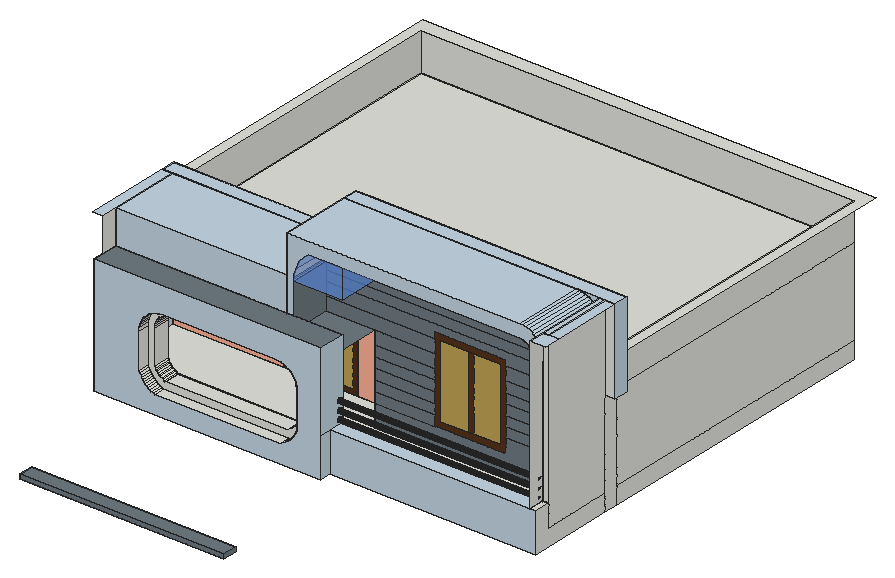
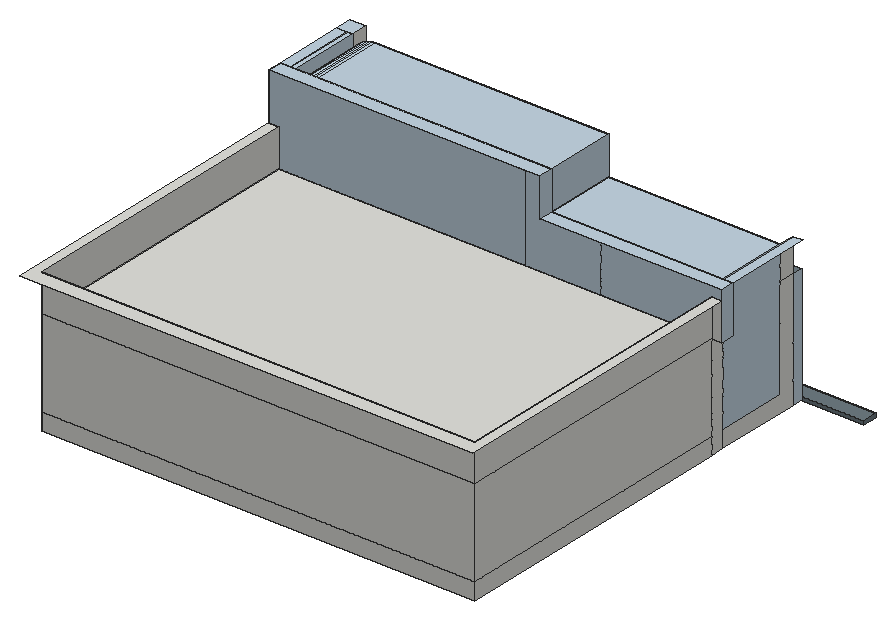
# SketchUp Ruby script. Lengths in inches.
U = 1.inch
M = Sketchup.active_model
def pt(a) = Geom::Point3d.new(a.map { |v| v * U })
def face(e, loops, mat)
  f = e.add_face(loops[0].map { |a| pt(a) })
  loops[1..].each { |l| e.add_face(l.map { |a| pt(a) }).erase! }
  f.material = f.back_material = mat if mat
  f
end
# faces: each face lists its corners as indices into pts; further lists are holes
def faces(e, pts, list, mat = nil) = list.each { |f| face(e, (f[0].is_a?(Array) ? f : [f]).map { |l| l.map { |i| pts[i] } }, mat) }
# xy, xz, yz: faces in a plane at the given z, y or x. An outline is a flat list of corners, or four numbers for a rectangle; further outlines are holes
def ring(l) = l.size == 4 ? [[l[0], l[1]], [l[2], l[1]], [l[2], l[3]], [l[0], l[3]]] : l.each_slice(2).to_a
def flat(e, list, mat, &to3) = list.each { |f| face(e, (f[0].is_a?(Array) ? f : [f]).map { |l| ring(l).map { |u, v| to3.(u, v) } }, mat) }
def xy(e, z, list, mat = nil) = flat(e, list, mat) { |x, y| [x, y, z] }
def xz(e, y, list, mat = nil) = flat(e, list, mat) { |x, z| [x, y, z] }
def yz(e, x, list, mat = nil) = flat(e, list, mat) { |y, z| [x, y, z] }
def lines(e, pts, list) = list.each { |a, b| e.add_line(pt(pts[a]), pt(pts[b])) }
# prism: a flat outline (further loops are holes) pulled along v
def prism(e, loops, v, mat = nil)
  f = face(e, loops, mat); d = Geom::Vector3d.new(v.map { |x| x * U })
  f.pushpull(f.normal.samedirection?(d) ? d.length : -d.length)
end
def box(e, o, s, mat = nil) = prism(e, [[o, [o[0] + s[0], o[1], o[2]], [o[0] + s[0], o[1] + s[1], o[2]], [o[0], o[1] + s[1], o[2]]]], [0, 0, s[2]], mat)
def at(x, y, z, deg = 0) = Geom::Transformation.translation(pt([x, y, z])) * Geom::Transformation.rotation(ORIGIN, Z_AXIS, deg.degrees)
def axes(o, x, y, z) = Geom::Transformation.new([*x, 0, *y, 0, *z, 0, *pt(o).to_a, 1])
def part(name) = M.definitions.add(name)
# library, detail: a bought-in or finely detailed component or shape, given as its bounding box
def library(name, o, s) = part(name).tap { |d| box(d.entities, o, s) }
def detail(e, o, s) = box(e.add_group.entities, o, s)
def put(e, d, t, mat = nil) = e.add_instance(d, t).tap { |i| i.material = mat if mat }
def group(e, t, mat = nil) = e.add_group.tap { |g| g.transformation = t; g.material = mat if mat }.entities
root = M.entities
M.materials.add("[Blinds Cloth Horizontal]").color = [192, 163, 85]
M.materials.add("[Blinds Wood Light]").color = [155, 100, 14]
M.materials.add("[Color B02]").color = [255, 178, 153]
M.materials.add("[Color M08]").color = [30, 30, 30]
M.materials.add("[Formica Speckled Grey]").color = [110, 123, 130]
M.materials.add("[Formica Speckled Grey]1").color = [94, 105, 111]
M.materials.add("[Terrazzo Light Blue]").color = [196, 214, 227]
M.materials.add("[Translucent Glass Blue]").color = [100, 149, 237]
M.materials["[Translucent Glass Blue]"].alpha = 0.5
M.materials.add("[Wood Veneer 01]").color = [81, 47, 25]
M.materials.add("[Wood Veneer 01]1").color = [86, 50, 26]
xy(root,238.16,[[0,105.19,19.68,134.14],[367.43,105.19,400.73,114.42],[367.43,114.42,400.73,134.14]])
xy(root,238.16,[[19.68,105.19,367.43,134.14]],"[Formica Speckled Grey]1")
xy(root,245.72,[[0,105.19,400.73,134.14]],"[Formica Speckled Grey]")
xy(root,330.6,[[460.73,414.17,460.73,454.3,19.68,454.3,19.68,482.57,868.09,482.57,868.09,454.3,539.55,454.3,539.55,414.17],[19.68,482.57,868.09,1063.55]])
xy(root,330.6,[[19.68,261.14,19.68,454.3,460.73,454.3,460.73,414.17,539.55,414.17,539.55,454.3,868.09,454.3,868.09,283.27,464.39,283.27,464.39,261.14]],"[Color B02]")
xy(root,363.72,[[19.68,315.125,832.87,315.125,832.87,394.0625,464.39,394.0625,464.39,454.3,19.68,454.3],[832.87,315.125,832.87,394.0625,464.39,394.0625,464.39,454.3,857.27,454.3,857.27,315.125],[857.27,315.125,857.52,454.3],[857.52,315.125,868.09,454.3],[237.18,454.3,383.16,482.57],
  [19.68,482.57,868.09,1063.55]])
xy(root,365.69,[[139.67,261.14,383.91,283.27]])
xy(root,379.22,[[142.77,283.27,381.06,315.125]])
xy(root,407.22,[[857.52,283.27,868.09,315.125]])
xy(root,407.78,[[464.39,283.27,857.52,315.125]],"[Terrazzo Light Blue]")
xy(root,415.4375,[[76.14,454.3,151.32,482.57]])
xy(root,498.17,[[153.41,283.27,376.34,315.125]])
xy(root,507,[[76.14,454.3,151.32,482.57]])
xy(root,511.69,[[153.41,261.14,376.34,283.27]])
xy(root,518.32,[[237.18,454.3,383.16,482.57]])
xy(root,535.72,[[356.14,315.125,369.45,315.125,369.45,394.0625,464.39,394.0625,464.39,454.3,356.14,454.3],[0,454.3,19.68,482.57],[868.09,454.3,887.77,482.57],[19.68,482.57,868.09,1063.55]])
xy(root,535.72,[[369.45,315.125,464.39,394.0625]],"[Formica Speckled Grey]")
xy(root,561.66,[[19.68,261.14,464.39,315.125]],"[Formica Speckled Grey]")
xy(root,609.41,[[0,482.57,19.68,482.57,19.68,1063.55,868.09,1063.55,868.09,482.57,887.77,482.57,887.77,1092.49,0,1092.49]])
xy(root,621.38,[[369.45,315.125,464.39,394.0625]],"[Translucent Glass Blue]")
xy(root,627.66,[[0,283.27,19.68,454.3],[19.68,315.125,356.14,454.3],[0,454.3,356.14,482.57]],"[Terrazzo Light Blue]")
xy(root,678.01,[[464.39,315.125,812.51,394.0625]],"[Formica Speckled Grey]")
xy(root,702.66,[[857.52,283.27,887.77,315.125],[356.14,315.125,812.51,454.3],[857.27,315.125,868.09,454.3],[868.09,315.125,887.77,454.3],[356.14,454.3,887.77,482.57]],"[Terrazzo Light Blue]")
xz(root,105.19,[[0,238.16,400.73,245.72]],"[Formica Speckled Grey]")
xz(root,134.14,[[0,238.16,400.73,245.72]],"[Formica Speckled Grey]")
xz(root,261.14,[[[19.68,330.6,464.39,561.66],[139.67,365.69,136.24,367.36,132.91,369.23,129.7,371.3,126.63,373.56,123.7,376,120.92,378.61,118.3,381.39,115.86,384.32,113.6,387.4,111.54,390.6,109.67,393.93,108,397.36,108,466.29,108.39,472.22,109.55,478.04,111.46,483.67,114.09,488.99,117.39,493.93,121.3,498.4,125.77,502.3125,130.7,505.61,136.03,508.24,141.66,510.15,147.48,511.31,153.41,511.69,376.34,511.69,381.85,511.33,387.27,510.26,392.5,508.48,397.45,506.04,402.05,502.97,406.2,499.33,409.84,495.18,412.91,490.58,415.35,485.63,417.125,480.4,418.2,474.98,418.57,469.47,418.57,400.35,416.87,396.51,414.93,392.79,412.73,389.22,410.3,385.79,407.65,382.54,404.78,379.48,401.72,376.61,398.47,373.96,395.04,371.53,391.47,369.33,387.75,367.39,383.91,365.69]]],"[Terrazzo Light Blue]")
xz(root,283.27,[[[139.67,365.69,383.91,365.69,387.75,367.39,391.47,369.33,395.04,371.53,398.47,373.96,401.72,376.61,404.78,379.48,407.65,382.54,410.3,385.79,412.73,389.22,414.93,392.79,416.87,396.51,418.57,400.35,418.57,469.47,418.2,474.98,417.125,480.4,415.35,485.63,412.91,490.58,409.84,495.18,406.2,499.33,402.05,502.97,397.45,506.04,392.5,508.48,387.27,510.26,381.85,511.33,376.34,511.69,153.41,511.69,147.48,511.31,141.66,510.15,136.03,508.24,130.7,505.61,125.77,502.3125,121.3,498.4,117.39,493.93,114.09,488.99,111.46,483.67,109.55,478.04,108.39,472.22,108,466.29,108,397.36,109.67,393.93,111.54,390.6,113.6,387.4,115.86,384.32,118.3,381.39,120.92,378.61,123.7,376,126.63,373.56,129.7,371.3,132.91,369.23,136.24,367.36],[142.77,379.22,142.51,379.35,139.9,380.82,137.38,382.44,134.97,384.21,132.67,386.13,130.49,388.18,128.4375,390.36,126.52,392.66,124.75,395.07,123.125,397.59,121.66,400.2,121.53,400.47,121.53,466.29,121.8,470.45,122.62,474.54,123.96,478.49,125.8,482.23,128.12,485.7,130.87,488.83,134,491.58,137.47,493.9,141.21,495.74,145.16,497.08,149.25,497.89,153.41,498.17,376.34,498.17,380.09,497.92,383.77,497.19,387.32,495.98,390.69,494.32,393.8125,492.24,396.63,489.76,399.11,486.94,401.19,483.82,402.85,480.45,404.06,476.9,404.79,473.22,405.04,469.47,405.04,403.2,404.68,402.38,403.15,399.47,401.4375,396.67,399.54,393.99,397.46,391.45,395.21,389.05,392.8125,386.8,390.27,384.72,387.59,382.82,384.79,381.11,381.875,379.58,381.06,379.22]]])
xz(root,283.27,[[464.39,330.6,868.09,330.6,868.09,407.22,857.52,407.22,857.52,407.78,464.39,407.78]],"[Terrazzo Light Blue]")
xz(root,315.125,[[[19.68,363.72,19.68,561.66,356.14,561.66,356.14,535.72,464.39,535.72,464.39,363.72],[142.77,379.22,381.06,379.22,381.875,379.58,384.79,381.11,387.59,382.82,390.27,384.72,392.8125,386.8,395.21,389.05,397.46,391.45,399.54,393.99,401.4375,396.67,403.15,399.47,404.68,402.38,405.04,403.2,405.04,469.47,404.79,473.22,404.06,476.9,402.85,480.45,401.19,483.82,399.11,486.94,396.63,489.76,393.8125,492.24,390.69,494.32,387.32,495.98,383.77,497.19,380.09,497.92,376.34,498.17,153.41,498.17,149.25,497.89,145.16,497.08,141.21,495.74,137.47,493.9,134,491.58,130.87,488.83,128.12,485.7,125.8,482.23,123.96,478.49,122.62,474.54,121.8,470.45,121.53,466.29,121.53,400.47,121.66,400.2,123.125,397.59,124.75,395.07,126.52,392.66,128.4375,390.36,130.49,388.18,132.67,386.13,134.97,384.21,137.38,382.44,139.9,380.82,142.51,379.35]],[464.39,363.72,832.87,407.78],[832.87,363.72,857.27,407.78],[857.27,363.72,857.52,407.22],[857.52,363.72,868.09,407.22],
  [857.27,407.22,857.52,407.78],[857.52,407.22,868.09,702.66],[857.52,657.65,857.52,702.66,857.27,702.66,857.27,661.46]])
xz(root,315.125,[[356.14,535.72,369.45,561.66],[369.45,535.72,464.39,561.66]],"[Formica Speckled Grey]")
xz(root,315.125,[[832.87,407.78,857.27,407.78,857.27,661.46,857.14,663.52,855.99,669.3,854.1,674.87,851.49,680.15,848.22,685.05,844.34,689.48,839.91,693.36,835.02,696.63,829.74,699.23,824.16,701.125,818.39,702.27,812.51,702.66,356.14,702.66,356.14,561.66,369.45,561.66,369.45,621.38,369.36,626.98,369.45,628.23,369.77,632.57,370.69,638.09,372.11,643.51,374.02,648.78,376.39,653.85,379.21,658.68,382.47,663.24,386.12,667.49,390.14,671.39,394.5,674.9,399.16,678.01,812.51,678.01,815.17,677.83,817.78,677.32,820.3,676.46,822.69,675.28,824.91,673.8,826.91,672.05,828.67,670.04,830.14,667.83,831.32,665.44,832.18,662.92,832.7,660.31,832.87,657.65],[19.68,561.66,356.14,627.66]],"[Terrazzo Light Blue]")
xz(root,315.125,[[369.45,621.38,464.39,621.38,464.39,678.01,399.16,678.01,394.5,674.9,390.14,671.39,386.12,667.49,382.47,663.24,379.21,658.68,376.39,653.85,374.02,648.78,372.11,643.51,370.69,638.09,369.77,632.57,369.45,628.23]],"[Translucent Glass Blue]")
xz(root,394.0625,[[369.45,621.38,369.45,628.23,369.36,626.98]])
xz(root,394.0625,[[594.64,420.01,647.18,561.5625],[658.36,420.01,710.7,561.5625]],"[Blinds Cloth Horizontal]")
xz(root,394.0625,[[464.39,363.72,832.87,363.72,832.87,435.72,722.29,435.72,722.29,408.41,583.04,408.41,583.04,427.0625,464.39,427.0625],[464.39,427.0625,583.04,447.625],[722.29,435.72,832.87,455.72],[464.39,447.625,583.04,468.1875],[722.29,455.72,832.87,475.72],
  [464.39,468.1875,583.04,488.75],[722.29,475.72,832.87,495.72],[464.39,488.75,583.04,509.3125],[722.29,495.72,832.87,515.72],[464.39,509.3125,583.04,535.72],
  [722.29,515.72,832.87,535.72],[369.45,535.72,583.04,561.8125],[722.29,535.72,832.87,561.8125],[369.45,561.8125,583.04,561.8125,583.04,573.16,722.29,573.16,722.29,561.8125,832.87,561.8125,832.87,587.9,369.45,587.9],[369.45,587.9,832.87,607.65],
  [369.45,607.65,832.87,607.65,832.87,631.96,464.39,631.96,464.39,621.38,369.45,621.38],[464.39,631.96,832.87,631.96,832.87,657.65,464.39,656.55],[464.39,656.55,832.87,657.65,832.7,660.31,832.18,662.92,831.32,665.44,830.14,667.83,828.67,670.04,826.91,672.05,824.91,673.8,822.69,675.28,820.3,676.46,817.78,677.32,815.17,677.83,812.51,678.01,464.39,678.01]],"[Formica Speckled Grey]")
xz(root,394.0625,[[[583.04,408.41,722.29,573.16],[594.64,420.01,710.7,561.5625]],[647.18,420.01,658.36,561.5625]],"[Wood Veneer 01]1")
xz(root,454.3,[[464.39,363.72,636.63,363.72,636.63,498.23,716.95,498.23,716.95,363.72,857.27,363.72,857.27,661.46,857.14,663.52,855.99,669.3,854.1,674.87,851.49,680.15,848.22,685.05,844.34,689.48,839.91,693.36,835.02,696.63,829.74,699.23,824.16,701.125,818.39,702.27,812.51,702.66,356.14,702.66,356.14,535.72,464.39,535.72],[857.27,363.72,857.52,535.72],[857.52,363.72,868.09,535.72],[857.27,535.72,857.52,535.72,857.52,657.65,857.27,661.46],[857.27,535.72,857.52,535.72,857.52,657.65,857.27,661.46],
  [857.52,535.72,868.09,535.72,868.09,702.66,857.27,702.66,857.27,661.46,857.52,657.65],[868.09,535.72,887.77,702.66]])
xz(root,454.3,[[246.5625,373.09,299.1,508.95],[310.17,373.09,373.78,508.95]],"[Blinds Cloth Horizontal]")
xz(root,454.3,[[643.85,413.07,671.92,491.01],[678.94,413.07,709.73,491.01],[83.73,423.03,110,499.41],[116.23,423.03,143.73,499.41]],"[Blinds Wood Light]")
xz(root,454.3,[[[19.68,363.72,237.18,363.72,237.18,518.32,383.16,518.32,383.16,363.72,464.39,363.72,464.39,535.72,356.14,535.72,356.14,627.66,19.68,627.66],[76.14,415.4375,151.32,507]]],"[Color B02]")
xz(root,454.3,[[0,535.72,19.68,627.66],[857.27,661.46,857.27,702.66,812.51,702.66,818.39,702.27,824.16,701.125,829.74,699.23,835.02,696.63,839.91,693.36,844.34,689.48,848.22,685.05,851.49,680.15,854.1,674.87,855.99,669.3,857.14,663.52]],"[Terrazzo Light Blue]")
xz(root,454.3,[[237.18,363.72,299.1,363.72,299.1,373.09,246.5625,373.09,246.5625,508.95,299.1,508.95,299.1,518.32,237.18,518.32],[299.1,363.72,310.17,373.09],[310.17,363.72,383.16,363.72,383.16,518.32,310.17,518.32,310.17,508.95,373.78,508.95,373.78,373.09,310.17,373.09],[[636.63,363.72,716.95,498.23],[643.85,413.07,709.73,491.01]],[299.1,373.09,310.17,508.95],
  [671.92,413.07,678.94,491.01],[[76.14,415.4375,151.32,507],[83.73,423.03,143.73,499.41]],[110,423.03,116.23,499.41],[299.1,508.95,310.17,518.32]],"[Wood Veneer 01]")
xz(root,482.57,[[19.68,330.6,868.09,363.72],[[19.68,363.72,19.68,535.72,868.09,535.72,868.09,363.72,383.16,363.72,383.16,518.32,237.18,518.32,237.18,363.72],[76.14,415.4375,151.32,507]],[0,535.72,19.68,609.41],[868.09,535.72,887.77,609.41]])
xz(root,482.57,[[19.68,535.72,19.68,609.41,0,609.41,0,627.66,237.18,627.66,237.18,535.72],[237.18,535.72,237.18,627.66,356.14,627.66,356.14,702.66,383.16,702.66,383.16,535.72],[383.16,535.72,383.16,702.66,887.77,702.66,887.77,609.41,868.09,609.41,868.09,535.72]],"[Terrazzo Light Blue]")
xz(root,1063.55,[[19.68,330.6,868.09,363.72],[19.68,363.72,868.09,535.72],[19.68,535.72,868.09,609.41]])
yz(root,0,[[105.19,238.16,134.14,245.72]],"[Formica Speckled Grey]")
yz(root,0,[[454.3,535.72,482.57,627.66]],"[Terrazzo Light Blue]")
yz(root,19.68,[[283.27,330.6,283.27,561.66,315.125,561.66,315.125,363.72,454.3,363.72,454.3,330.6],[454.3,330.6,482.57,535.72],[482.57,330.6,1063.55,363.72],[482.57,363.72,1063.55,535.72],[482.57,535.72,1063.55,609.41],
  [283.27,561.66,315.125,627.66]])
yz(root,19.68,[[261.14,330.6,283.27,561.66],[315.125,363.72,454.3,627.66]],"[Terrazzo Light Blue]")
yz(root,76.14,[[454.3,415.4375,482.57,507]])
yz(root,108,[[261.14,397.36,283.27,466.29]])
yz(root,121.53,[[283.27,400.47,315.125,466.29]])
yz(root,151.32,[[454.3,415.4375,482.57,507]])
yz(root,237.18,[[454.3,363.72,482.57,518.32]])
yz(root,356.14,[[315.125,535.72,454.3,627.66]])
yz(root,356.14,[[315.125,627.66,454.3,702.66],[454.3,627.66,482.57,702.66]],"[Terrazzo Light Blue]")
yz(root,369.45,[[315.125,535.72,394.0625,621.38]],"[Formica Speckled Grey]")
yz(root,369.45,[[315.125,621.38,394.0625,628.23]],"[Translucent Glass Blue]")
yz(root,383.16,[[454.3,363.72,482.57,518.32]])
yz(root,400.73,[[105.19,238.16,134.14,245.72]],"[Formica Speckled Grey]")
yz(root,405.04,[[283.27,403.2,315.125,469.47]])
yz(root,418.57,[[261.14,400.35,283.27,469.47]])
yz(root,464.39,[[305.4375,413.46,304.43,413.6,303.5,413.98,302.7,414.6,302.08,415.4,301.69,416.34,301.5625,417.34,301.69,418.34,302.08,419.28,302.7,420.08,303.5,420.7,304.43,421.08,305.4375,421.21,306.44,421.08,307.375,420.7,308.18,420.08,308.79,419.28,309.18,418.34,309.3125,417.34,309.18,416.34,308.79,415.4,308.18,414.6,307.375,413.98,306.44,413.6],[305.4375,429.65,304.43,429.78,303.5,430.17,302.7,430.79,302.08,431.59,301.69,432.52,301.5625,433.53,301.69,434.53,302.08,435.46,302.7,436.27,303.5,436.88,304.43,437.27,305.4375,437.4,306.44,437.27,307.375,436.88,308.18,436.27,308.79,435.46,309.18,434.53,309.3125,433.53,309.18,432.52,308.79,431.59,308.18,430.79,307.375,430.17,306.44,429.78],[305.4375,447.21,304.43,447.35,303.5,447.73,302.7,448.35,302.08,449.15,301.69,450.09,301.5625,451.09,301.69,452.09,302.08,453.03,302.7,453.83,303.5,454.45,304.43,454.83,305.4375,454.96,306.44,454.83,307.375,454.45,308.18,453.83,308.79,453.03,309.18,452.09,309.3125,451.09,309.18,450.09,308.79,449.15,308.18,448.35,307.375,447.73,306.44,447.35]])
yz(root,464.39,[[261.14,330.6,283.27,407.22],[394.0625,363.72,454.3,535.72],[[261.14,407.22,283.27,407.22,283.27,407.78,315.125,407.78,315.125,561.66,261.14,561.66],[305.4375,413.46,304.43,413.6,303.5,413.98,302.7,414.6,302.08,415.4,301.69,416.34,301.5625,417.34,301.69,418.34,302.08,419.28,302.7,420.08,303.5,420.7,304.43,421.08,305.4375,421.21,306.44,421.08,307.375,420.7,308.18,420.08,308.79,419.28,309.18,418.34,309.3125,417.34,309.18,416.34,308.79,415.4,308.18,414.6,307.375,413.98,306.44,413.6],[305.4375,429.65,304.43,429.78,303.5,430.17,302.7,430.79,302.08,431.59,301.69,432.52,301.5625,433.53,301.69,434.53,302.08,435.46,302.7,436.27,303.5,436.88,304.43,437.27,305.4375,437.4,306.44,437.27,307.375,436.88,308.18,436.27,308.79,435.46,309.18,434.53,309.3125,433.53,309.18,432.52,308.79,431.59,308.18,430.79,307.375,430.17,306.44,429.78],[305.4375,447.21,304.43,447.35,303.5,447.73,302.7,448.35,302.08,449.15,301.69,450.09,301.5625,451.09,301.69,452.09,302.08,453.03,302.7,453.83,303.5,454.45,304.43,454.83,305.4375,454.96,306.44,454.83,307.375,454.45,308.18,453.83,308.79,453.03,309.18,452.09,309.3125,451.09,309.18,450.09,308.79,449.15,308.18,448.35,307.375,447.73,306.44,447.35]]],"[Terrazzo Light Blue]")
yz(root,464.39,[[315.125,621.38,394.0625,678.01]],"[Translucent Glass Blue]")
yz(root,832.87,[[315.125,363.72,394.0625,407.22]])
yz(root,832.87,[[315.125,407.22,394.0625,657.65]],"[Formica Speckled Grey]")
yz(root,857.27,[[315.125,363.72,454.3,702.66]],"[Terrazzo Light Blue]")
yz(root,857.52,[[315.125,363.72,454.3,657.65],[283.27,407.22,315.125,407.78],[[283.27,407.78,315.125,702.66],[305.4375,447.21,304.43,447.35,303.5,447.73,302.7,448.35,302.08,449.15,301.69,450.09,301.5625,451.09,301.69,452.09,302.08,453.03,302.7,453.83,303.5,454.45,304.43,454.83,305.4375,454.96,306.44,454.83,307.375,454.45,308.18,453.83,308.79,453.03,309.18,452.09,309.3125,451.09,309.18,450.09,308.79,449.15,308.18,448.35,307.375,447.73,306.44,447.35],[305.4375,429.65,304.43,429.78,303.5,430.17,302.7,430.79,302.08,431.59,301.69,432.52,301.5625,433.53,301.69,434.53,302.08,435.46,302.7,436.27,303.5,436.88,304.43,437.27,305.4375,437.4,306.44,437.27,307.375,436.88,308.18,436.27,308.79,435.46,309.18,434.53,309.3125,433.53,309.18,432.52,308.79,431.59,308.18,430.79,307.375,430.17,306.44,429.78],[305.4375,413.46,304.43,413.6,303.5,413.98,302.7,414.6,302.08,415.4,301.69,416.34,301.5625,417.34,301.69,418.34,302.08,419.28,302.7,420.08,303.5,420.7,304.43,421.08,305.4375,421.21,306.44,421.08,307.375,420.7,308.18,420.08,308.79,419.28,309.18,418.34,309.3125,417.34,309.18,416.34,308.79,415.4,308.18,414.6,307.375,413.98,306.44,413.6]]])
yz(root,868.09,[[283.27,330.6,454.3,330.6,454.3,363.72,315.125,363.72,315.125,407.22,283.27,407.22],[454.3,330.6,482.57,535.72],[482.57,330.6,1063.55,363.72],[315.125,363.72,454.3,702.66],[482.57,363.72,1063.55,535.72],
  [482.57,535.72,1063.55,609.41]])
yz(root,887.77,[[454.3,535.72,482.57,702.66]],"[Terrazzo Light Blue]")
p = [[139.67,283.27,365.69],[136.24,283.27,367.36],[136.24,261.14,367.36],[139.67,261.14,365.69],[387.75,283.27,367.39],[383.91,283.27,365.69],
  [383.91,261.14,365.69],[387.75,261.14,367.39],[132.91,283.27,369.23],[132.91,261.14,369.23],[391.47,283.27,369.33],[391.47,261.14,369.33],
  [129.7,283.27,371.3],[129.7,261.14,371.3],[395.04,283.27,371.53],[395.04,261.14,371.53],[126.63,283.27,373.56],[126.63,261.14,373.56],
  [398.47,283.27,373.96],[398.47,261.14,373.96],[123.7,283.27,376],[123.7,261.14,376],[401.72,283.27,376.61],[401.72,261.14,376.61],
  [120.92,283.27,378.61],[120.92,261.14,378.61],[404.78,283.27,379.48],[404.78,261.14,379.48],[118.3,283.27,381.39],[118.3,261.14,381.39],
  [142.51,283.27,379.35],[142.77,283.27,379.22],[142.77,315.125,379.22],[142.51,315.125,379.35],[381.06,283.27,379.22],[381.875,283.27,379.58],
  [381.875,315.125,379.58],[381.06,315.125,379.22],[139.9,283.27,380.82],[139.9,315.125,380.82],[407.65,283.27,382.54],[407.65,261.14,382.54],
  [384.79,283.27,381.11],[384.79,315.125,381.11],[137.38,283.27,382.44],[137.38,315.125,382.44],[387.59,283.27,382.82],[387.59,315.125,382.82],
  [115.86,283.27,384.32],[115.86,261.14,384.32],[134.97,283.27,384.21],[134.97,315.125,384.21],[410.3,283.27,385.79],[410.3,261.14,385.79],
  [390.27,283.27,384.72],[390.27,315.125,384.72],[132.67,283.27,386.13],[132.67,315.125,386.13],[113.6,283.27,387.4],[113.6,261.14,387.4],
  [392.8125,283.27,386.8],[392.8125,315.125,386.8],[412.73,283.27,389.22],[412.73,261.14,389.22],[130.49,283.27,388.18],[130.49,315.125,388.18],
  [395.21,283.27,389.05],[395.21,315.125,389.05],[111.54,283.27,390.6],[111.54,261.14,390.6],[128.4375,283.27,390.36],[128.4375,315.125,390.36],
  [397.46,283.27,391.45],[397.46,315.125,391.45],[414.93,283.27,392.79],[414.93,261.14,392.79],[126.52,283.27,392.66],[126.52,315.125,392.66],
  [109.67,283.27,393.93],[109.67,261.14,393.93],[399.54,283.27,393.99],[399.54,315.125,393.99],[124.75,283.27,395.07],[124.75,315.125,395.07],
  [416.87,283.27,396.51],[416.87,261.14,396.51],[108,283.27,397.36],[108,261.14,397.36],[401.4375,283.27,396.67],[401.4375,315.125,396.67],
  [123.125,283.27,397.59],[123.125,315.125,397.59],[418.57,283.27,400.35],[418.57,261.14,400.35],[403.15,283.27,399.47],[403.15,315.125,399.47],
  [121.66,283.27,400.2],[121.66,315.125,400.2],[404.68,283.27,402.38],[404.68,315.125,402.38],[121.53,283.27,400.47],[121.53,315.125,400.47],
  [405.04,283.27,403.2],[405.04,315.125,403.2],[464.39,304.43,413.6],[464.39,305.4375,413.46],[857.52,305.4375,413.46],[857.52,304.43,413.6],
  [464.39,306.44,413.6],[857.52,306.44,413.6],[464.39,303.5,413.98],[857.52,303.5,413.98],[464.39,307.375,413.98],[857.52,307.375,413.98],
  [464.39,302.7,414.6],[857.52,302.7,414.6],[464.39,308.18,414.6],[857.52,308.18,414.6],[464.39,302.08,415.4],[857.52,302.08,415.4],
  [464.39,308.79,415.4],[857.52,308.79,415.4],[464.39,301.69,416.34],[857.52,301.69,416.34],[464.39,309.18,416.34],[857.52,309.18,416.34],
  [464.39,301.5625,417.34],[857.52,301.5625,417.34],[464.39,309.3125,417.34],[857.52,309.3125,417.34],[464.39,301.69,418.34],[857.52,301.69,418.34],
  [464.39,309.18,418.34],[857.52,309.18,418.34],[464.39,302.08,419.28],[857.52,302.08,419.28],[464.39,308.79,419.28],[857.52,308.79,419.28],
  [464.39,302.7,420.08],[857.52,302.7,420.08],[464.39,308.18,420.08],[857.52,308.18,420.08],[464.39,303.5,420.7],[857.52,303.5,420.7],
  [464.39,307.375,420.7],[857.52,307.375,420.7],[464.39,304.43,421.08],[857.52,304.43,421.08],[464.39,306.44,421.08],[857.52,306.44,421.08],
  [464.39,305.4375,421.21],[857.52,305.4375,421.21],[464.39,304.43,429.78],[464.39,305.4375,429.65],[857.52,305.4375,429.65],[857.52,304.43,429.78],
  [464.39,306.44,429.78],[857.52,306.44,429.78],[464.39,303.5,430.17],[857.52,303.5,430.17],[464.39,307.375,430.17],[857.52,307.375,430.17],
  [464.39,302.7,430.79],[857.52,302.7,430.79],[464.39,308.18,430.79],[857.52,308.18,430.79],[464.39,302.08,431.59],[857.52,302.08,431.59],
  [464.39,308.79,431.59],[857.52,308.79,431.59],[464.39,301.69,432.52],[857.52,301.69,432.52],[464.39,309.18,432.52],[857.52,309.18,432.52],
  [464.39,301.5625,433.53],[857.52,301.5625,433.53],[464.39,309.3125,433.53],[857.52,309.3125,433.53],[464.39,301.69,434.53],[857.52,301.69,434.53],
  [464.39,309.18,434.53],[857.52,309.18,434.53],[464.39,302.08,435.46],[857.52,302.08,435.46],[464.39,308.79,435.46],[857.52,308.79,435.46],
  [464.39,302.7,436.27],[857.52,302.7,436.27],[464.39,308.18,436.27],[857.52,308.18,436.27],[464.39,303.5,436.88],[857.52,303.5,436.88],
  [464.39,307.375,436.88],[857.52,307.375,436.88],[464.39,304.43,437.27],[857.52,304.43,437.27],[464.39,306.44,437.27],[857.52,306.44,437.27],
  [464.39,305.4375,437.4],[857.52,305.4375,437.4],[464.39,304.43,447.35],[464.39,305.4375,447.21],[857.52,305.4375,447.21],[857.52,304.43,447.35],
  [464.39,306.44,447.35],[857.52,306.44,447.35],[464.39,303.5,447.73],[857.52,303.5,447.73],[464.39,307.375,447.73],[857.52,307.375,447.73],
  [464.39,302.7,448.35],[857.52,302.7,448.35],[464.39,308.18,448.35],[857.52,308.18,448.35],[464.39,302.08,449.15],[857.52,302.08,449.15],
  [464.39,308.79,449.15],[857.52,308.79,449.15],[464.39,301.69,450.09],[857.52,301.69,450.09],[464.39,309.18,450.09],[857.52,309.18,450.09],
  [464.39,301.5625,451.09],[857.52,301.5625,451.09],[464.39,309.3125,451.09],[857.52,309.3125,451.09],[464.39,301.69,452.09],[857.52,301.69,452.09],
  [464.39,309.18,452.09],[857.52,309.18,452.09],[464.39,302.08,453.03],[857.52,302.08,453.03],[464.39,308.79,453.03],[857.52,308.79,453.03],
  [464.39,302.7,453.83],[857.52,302.7,453.83],[464.39,308.18,453.83],[857.52,308.18,453.83],[464.39,303.5,454.45],[857.52,303.5,454.45],
  [464.39,307.375,454.45],[857.52,307.375,454.45],[464.39,304.43,454.83],[857.52,304.43,454.83],[464.39,306.44,454.83],[857.52,306.44,454.83],
  [464.39,305.4375,454.96],[857.52,305.4375,454.96],[108,283.27,466.29],[108.39,283.27,472.22],[108.39,261.14,472.22],[108,261.14,466.29],
  [121.8,283.27,470.45],[121.53,283.27,466.29],[121.53,315.125,466.29],[121.8,315.125,470.45],[418.2,283.27,474.98],[418.57,283.27,469.47],
  [418.57,261.14,469.47],[418.2,261.14,474.98],[405.04,283.27,469.47],[404.79,283.27,473.22],[404.79,315.125,473.22],[405.04,315.125,469.47],
  [122.62,283.27,474.54],[122.62,315.125,474.54],[109.55,283.27,478.04],[109.55,261.14,478.04],[404.06,283.27,476.9],[404.06,315.125,476.9],
  [123.96,283.27,478.49],[123.96,315.125,478.49],[417.125,283.27,480.4],[417.125,261.14,480.4],[402.85,283.27,480.45],[402.85,315.125,480.45],
  [111.46,283.27,483.67],[111.46,261.14,483.67],[125.8,283.27,482.23],[125.8,315.125,482.23],[415.35,283.27,485.63],[415.35,261.14,485.63],
  [401.19,283.27,483.82],[401.19,315.125,483.82],[128.12,283.27,485.7],[128.12,315.125,485.7],[114.09,283.27,488.99],[114.09,261.14,488.99],
  [399.11,283.27,486.94],[399.11,315.125,486.94],[412.91,283.27,490.58],[412.91,261.14,490.58],[130.87,283.27,488.83],[130.87,315.125,488.83],
  [396.63,283.27,489.76],[396.63,315.125,489.76],[134,283.27,491.58],[134,315.125,491.58],[117.39,283.27,493.93],[117.39,261.14,493.93],
  [393.8125,283.27,492.24],[393.8125,315.125,492.24],[409.84,283.27,495.18],[409.84,261.14,495.18],[137.47,283.27,493.9],[137.47,315.125,493.9],
  [390.69,283.27,494.32],[390.69,315.125,494.32],[121.3,283.27,498.4],[121.3,261.14,498.4],[141.21,283.27,495.74],[141.21,315.125,495.74],
  [387.32,283.27,495.98],[387.32,315.125,495.98],[406.2,283.27,499.33],[406.2,261.14,499.33],[145.16,283.27,497.08],[145.16,315.125,497.08],
  [383.77,283.27,497.19],[383.77,315.125,497.19],[149.25,283.27,497.89],[149.25,315.125,497.89],[380.09,283.27,497.92],[380.09,315.125,497.92],
  [153.41,283.27,498.17],[153.41,315.125,498.17],[376.34,283.27,498.17],[376.34,315.125,498.17],[125.77,283.27,502.3125],[125.77,261.14,502.3125],
  [402.05,283.27,502.97],[402.05,261.14,502.97],[130.7,283.27,505.61],[130.7,261.14,505.61],[397.45,283.27,506.04],[397.45,261.14,506.04],
  [136.03,283.27,508.24],[136.03,261.14,508.24],[392.5,283.27,508.48],[392.5,261.14,508.48],[141.66,283.27,510.15],[141.66,261.14,510.15],
  [387.27,283.27,510.26],[387.27,261.14,510.26],[147.48,283.27,511.31],[147.48,261.14,511.31],[381.85,283.27,511.33],[381.85,261.14,511.33],
  [153.41,283.27,511.69],[153.41,261.14,511.69],[376.34,283.27,511.69],[376.34,261.14,511.69],[369.45,394.0625,621.38],[369.36,394.0625,626.98],
  [369.36,315.125,626.98],[369.45,315.125,621.38],[369.45,394.0625,628.23],[369.45,315.125,628.23],[832.7,394.0625,660.31],[832.87,394.0625,657.65],
  [832.87,315.125,657.65],[832.7,315.125,660.31],[857.14,454.3,663.52],[857.14,315.125,663.52],[857.27,315.125,661.46],[857.52,315.125,657.65],
  [857.52,454.3,657.65],[857.27,454.3,661.46],[832.18,394.0625,662.92],[832.18,315.125,662.92],[831.32,394.0625,665.44],[831.32,315.125,665.44],
  [855.99,454.3,669.3],[855.99,315.125,669.3],[830.14,394.0625,667.83],[830.14,315.125,667.83],[828.67,394.0625,670.04],[828.67,315.125,670.04],
  [854.1,454.3,674.87],[854.1,315.125,674.87],[826.91,394.0625,672.05],[826.91,315.125,672.05],[824.91,394.0625,673.8],[824.91,315.125,673.8],
  [822.69,394.0625,675.28],[822.69,315.125,675.28],[851.49,454.3,680.15],[851.49,315.125,680.15],[820.3,394.0625,676.46],[820.3,315.125,676.46],
  [817.78,394.0625,677.32],[817.78,315.125,677.32],[815.17,394.0625,677.83],[815.17,315.125,677.83],[812.51,394.0625,678.01],[812.51,315.125,678.01],
  [848.22,454.3,685.05],[848.22,315.125,685.05],[844.34,454.3,689.48],[844.34,315.125,689.48],[839.91,454.3,693.36],[839.91,315.125,693.36],
  [835.02,454.3,696.63],[835.02,315.125,696.63],[829.74,454.3,699.23],[829.74,315.125,699.23],[824.16,454.3,701.125],[824.16,315.125,701.125],
  [818.39,454.3,702.27],[818.39,315.125,702.27],[812.51,454.3,702.66],[812.51,315.125,702.66],[112.95,454.3,294.68],[112.95,482.57,294.68],
  [61.14,454.3,294.68],[61.14,482.57,294.68],[258.72,454.3,279.81],[258.72,482.57,279.81],[177.29,454.3,279.81],[177.29,482.57,279.81],
  [411.43,454.3,279.11],[411.43,482.57,279.11],[328.38,454.3,279.11],[328.38,482.57,279.11],[669.05,454.3,300.55],[669.05,482.57,300.55],
  [764.12,454.3,300.55],[764.12,482.57,300.55],[464.39,394.0625,406.5],[583.04,394.0625,406.5]]
faces(root,p,[[0,1,2,3],[4,5,6,7],[1,8,9,2],[10,4,7,11],[8,12,13,9],[14,10,11,15],[12,16,17,13],[18,14,15,19],
  [16,20,21,17],[22,18,19,23],[20,24,25,21],[26,22,23,27],[24,28,29,25],[30,31,32,33],[34,35,36,37],[38,30,33,39],
  [40,26,27,41],[35,42,43,36],[44,38,39,45],[42,46,47,43],[28,48,49,29],[50,44,45,51],[52,40,41,53],[46,54,55,47],
  [56,50,51,57],[48,58,59,49],[54,60,61,55],[62,52,53,63],[64,56,57,65],[60,66,67,61],[58,68,69,59],[70,64,65,71],
  [66,72,73,67],[74,62,63,75],[76,70,71,77],[68,78,79,69],[72,80,81,73],[82,76,77,83],[84,74,75,85],[78,86,87,79],
  [80,88,89,81],[90,82,83,91],[92,84,85,93],[88,94,95,89],[96,90,91,97],[94,98,99,95],[100,96,97,101],[98,102,103,99],
  [248,249,250,251],[252,253,254,255],[256,257,258,259],[260,261,262,263],[264,252,255,265],[249,266,267,250],[261,268,269,262],[270,264,265,271],
  [272,256,259,273],[268,274,275,269],[266,276,277,267],[278,270,271,279],[280,272,273,281],[274,282,283,275],[284,278,279,285],[276,286,287,277],
  [282,288,289,283],[290,280,281,291],[292,284,285,293],[288,294,295,289],[296,292,293,297],[286,298,299,287],[294,300,301,295],[302,290,291,303],
  [304,296,297,305],[300,306,307,301],[298,308,309,299],[310,304,305,311],[306,312,313,307],[314,302,303,315],[316,310,311,317],[312,318,319,313],
  [320,316,317,321],[318,322,323,319],[324,320,321,325],[322,326,327,323],[308,328,329,309],[330,314,315,331],[328,332,333,329],[334,330,331,335],
  [332,336,337,333],[338,334,335,339],[336,340,341,337],[342,338,339,343],[340,344,345,341],[346,342,343,347],[344,348,349,345],[350,346,347,351],
  [352,353,354,355],[353,356,357,354]])
faces(root,p,[[104,105,106,107],[105,108,109,106],[110,104,107,111],[108,112,113,109],[114,110,111,115],[112,116,117,113],[118,114,115,119],[116,120,121,117],
  [122,118,119,123],[120,124,125,121],[126,122,123,127],[124,128,129,125],[130,126,127,131],[128,132,133,129],[134,130,131,135],[132,136,137,133],
  [138,134,135,139],[136,140,141,137],[142,138,139,143],[140,144,145,141],[146,142,143,147],[144,148,149,145],[150,146,147,151],[148,150,151,149],
  [152,153,154,155],[153,156,157,154],[158,152,155,159],[156,160,161,157],[162,158,159,163],[160,164,165,161],[166,162,163,167],[164,168,169,165],
  [170,166,167,171],[168,172,173,169],[174,170,171,175],[172,176,177,173],[178,174,175,179],[176,180,181,177],[182,178,179,183],[180,184,185,181],
  [186,182,183,187],[184,188,189,185],[190,186,187,191],[188,192,193,189],[194,190,191,195],[192,196,197,193],[198,194,195,199],[196,198,199,197],
  [200,201,202,203],[201,204,205,202],[206,200,203,207],[204,208,209,205],[210,206,207,211],[208,212,213,209],[214,210,211,215],[212,216,217,213],
  [218,214,215,219],[216,220,221,217],[222,218,219,223],[220,224,225,221],[226,222,223,227],[224,228,229,225],[230,226,227,231],[228,232,233,229],
  [234,230,231,235],[232,236,237,233],[238,234,235,239],[236,240,241,237],[242,238,239,243],[240,244,245,241],[246,242,243,247],[244,246,247,245]],"[Color M08]")
faces(root,p,[[358,359,360,361],[368,358,361,369],[370,368,369,371],[374,370,371,375],[376,374,375,377],[380,376,377,381],[382,380,381,383],[384,382,383,385],
  [388,384,385,389],[390,388,389,391],[392,390,391,393],[394,392,393,395]],"[Formica Speckled Grey]")
faces(root,p,[[362,363,364,365,366,367],[372,373,363,362],[378,379,373,372],[386,387,379,378],[396,397,387,386],[398,399,397,396],[400,401,399,398],[402,403,401,400],
  [404,405,403,402],[406,407,405,404],[408,409,407,406],[410,411,409,408]],"[Terrazzo Light Blue]")
lines(root,p,[[412,413],[414,415],[416,417],[418,419],[420,421],[422,423],[424,425],[426,427],[428,429]])
